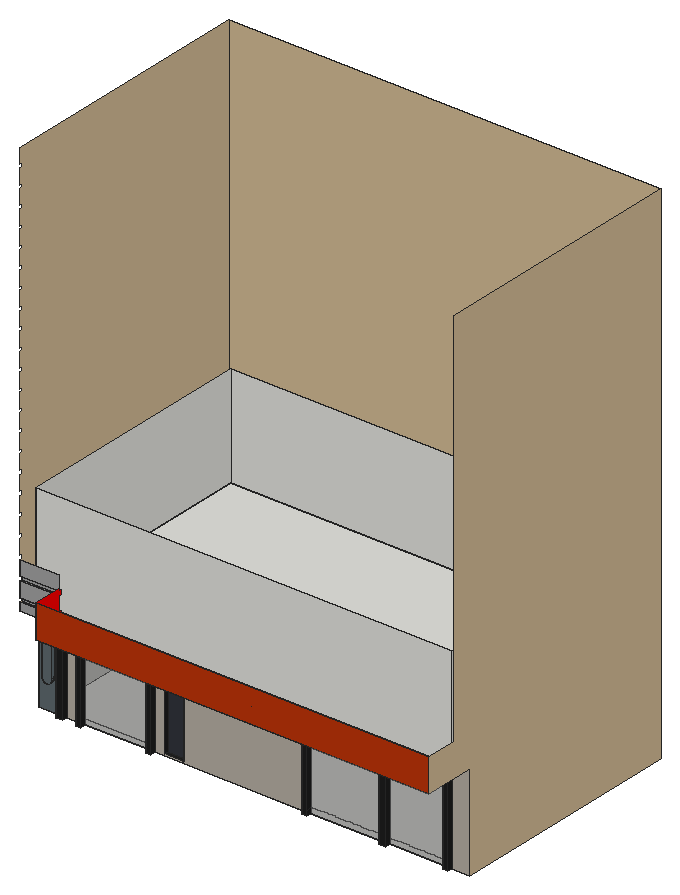
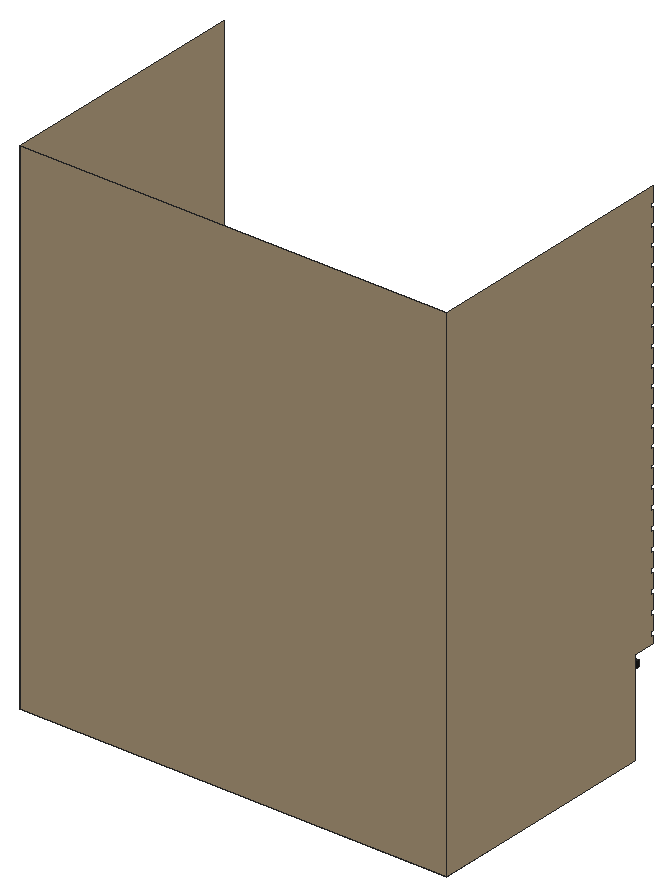
# SketchUp Ruby script. Lengths in inches.
U = 1.inch
M = Sketchup.active_model
def pt(a) = Geom::Point3d.new(a.map { |v| v * U })
def face(e, loops, mat)
  f = e.add_face(loops[0].map { |a| pt(a) })
  loops[1..].each { |l| e.add_face(l.map { |a| pt(a) }).erase! }
  f.material = f.back_material = mat if mat
  f
end
# faces: each face lists its corners as indices into pts; further lists are holes
def faces(e, pts, list, mat = nil) = list.each { |f| face(e, (f[0].is_a?(Array) ? f : [f]).map { |l| l.map { |i| pts[i] } }, mat) }
# xy, xz, yz: faces in a plane at the given z, y or x. An outline is a flat list of corners, or four numbers for a rectangle; further outlines are holes
def ring(l) = l.size == 4 ? [[l[0], l[1]], [l[2], l[1]], [l[2], l[3]], [l[0], l[3]]] : l.each_slice(2).to_a
def flat(e, list, mat, &to3) = list.each { |f| face(e, (f[0].is_a?(Array) ? f : [f]).map { |l| ring(l).map { |u, v| to3.(u, v) } }, mat) }
def xy(e, z, list, mat = nil) = flat(e, list, mat) { |x, y| [x, y, z] }
def xz(e, y, list, mat = nil) = flat(e, list, mat) { |x, z| [x, y, z] }
def yz(e, x, list, mat = nil) = flat(e, list, mat) { |y, z| [x, y, z] }
def lines(e, pts, list) = list.each { |a, b| e.add_line(pt(pts[a]), pt(pts[b])) }
# prism: a flat outline (further loops are holes) pulled along v
def prism(e, loops, v, mat = nil)
  f = face(e, loops, mat); d = Geom::Vector3d.new(v.map { |x| x * U })
  f.pushpull(f.normal.samedirection?(d) ? d.length : -d.length)
end
def box(e, o, s, mat = nil) = prism(e, [[o, [o[0] + s[0], o[1], o[2]], [o[0] + s[0], o[1] + s[1], o[2]], [o[0], o[1] + s[1], o[2]]]], [0, 0, s[2]], mat)
def at(x, y, z, deg = 0) = Geom::Transformation.translation(pt([x, y, z])) * Geom::Transformation.rotation(ORIGIN, Z_AXIS, deg.degrees)
def axes(o, x, y, z) = Geom::Transformation.new([*x, 0, *y, 0, *z, 0, *pt(o).to_a, 1])
def part(name) = M.definitions.add(name)
# library, detail: a bought-in or finely detailed component or shape, given as its bounding box
def library(name, o, s) = part(name).tap { |d| box(d.entities, o, s) }
def detail(e, o, s) = box(e.add_group.entities, o, s)
def put(e, d, t, mat = nil) = e.add_instance(d, t).tap { |i| i.material = mat if mat }
def group(e, t, mat = nil) = e.add_group.tap { |g| g.transformation = t; g.material = mat if mat }.entities
root = M.entities
M.materials.add("[0020_Red]").color = [255, 0, 0]
M.materials.add("[Blacktop New]").color = [30, 30, 30]
M.materials.add("[Formica Beige]").color = [211, 187, 149]
M.materials.add("[Formica Laminate Dark]").color = [50, 53, 60]
M.materials.add("[Formica Speckled Grey]").color = [94, 105, 111]
M.materials.add("[Modern Siding]1").color = [191, 52, 9]
M.materials.add("[Pavers Flagstone Gray]").color = [162, 162, 162]
M.materials.add("[Stone Masonry Multi]").color = [182, 175, 164]
M.materials.add("[Translucent Glass Gray]").color = [128, 128, 128]
M.materials["[Translucent Glass Gray]"].alpha = 0.5
M.materials.add("[Wood Veneer 01]").color = [120, 70, 37]
xy(root,0,[[[48.29,57,48.29,63,0,63,0,342.4375,506.625,342.4375,506.625,63,485.22,63,485.22,57,479.22,57,479.22,63,411.96,63,411.96,57,404.66,57,404.66,63,320.21,63,320.21,57,314.21,57,314.21,63,136.16,63,136.16,57,130.16,57,130.16,63,54.29,63,54.29,57],[9,72,497.625,333.4375]],[24.71,57,33.0625,63],[9,72,497.625,333.4375]])
xy(root,1.93,[[147.93,63,170.18,68.3125]],"[Blacktop New]")
xy(root,97.39,[[0,57,24.71,63]],"[Blacktop New]")
xy(root,99.6875,[[320.21,57,404.66,63],[411.96,57,479.22,63]],"[Blacktop New]")
xy(root,103.25,[[54.29,57,130.16,63]],"[Blacktop New]")
xy(root,105.58,[[0,57,33.0625,63]],"[Blacktop New]")
xy(root,105.6875,[[314.21,57,485.22,63]])
xy(root,109.25,[[48.29,57,136.16,63]],"[Blacktop New]")
xy(root,110.37,[[147.93,63,170.18,68.3125]],"[Blacktop New]")
xy(root,112.65,[[45.0625,3,45.0625,36,0,36,0,63,506.625,63,506.625,3]],"[Wood Veneer 01]")
xy(root,120,[[9,48,497.625,333.4375]])
xy(root,121.8125,[[0,36,45.0625,39]],"[Pavers Flagstone Gray]")
xy(root,126.82,[[0,36,45.0625,39]],"[Pavers Flagstone Gray]")
xy(root,144.1875,[[0,36,45.0625,39]],"[Pavers Flagstone Gray]")
xy(root,149.2,[[0,36,45.0625,39]],"[Pavers Flagstone Gray]")
xz(root,3,[[45.0625,112.65,506.625,151.96]],"[Modern Siding]1")
xz(root,36,[[0,112.65,45.0625,121.8125],[0,126.82,45.0625,144.1875],[0,149.2,45.0625,166.5625]],"[Pavers Flagstone Gray]")
xz(root,39,[[0,121.8125,45.0625,126.82],[0,144.1875,45.0625,149.2]],"[Pavers Flagstone Gray]")
xz(root,48,[[9,120,497.625,240]])
xz(root,57,[[24.71,0,33.0625,0,33.0625,105.58,0,105.58,0,97.39,24.71,97.39],[48.29,0,54.29,0,54.29,103.25,130.16,103.25,130.16,0,136.16,0,136.16,109.25,48.29,109.25],[314.21,0,320.21,0,320.21,99.6875,479.22,99.6875,479.22,0,485.22,0,485.22,105.6875,314.21,105.6875],[404.66,0,411.96,99.6875]],"[Blacktop New]")
xz(root,60,[[11.84,29.86,13.68,30.13,15.37,30.92,16.76,32.17,17.72,33.76,18.12,35.28,18.12,84,17.9,85.63,17.28,87.14,16.28,88.44,14.98,89.44,13.46,90.07,11.84,90.28,10.21,90.07,8.7,89.44,7.4,88.44,6.4,87.14,5.77,85.63,5.56,84,5.56,35.28,5.95,33.76,6.92,32.17,8.3,30.92,9.99,30.13]],"[Formica Speckled Grey]")
xz(root,63,[[24.71,0,24.71,97.39,0,97.39,0,105.58,33.0625,105.58,33.0625,0],[5.56,35.28,5.56,37.43,5.48,35.57],[18.12,35.28,18.19,35.57,18.12,37.43]])
xz(root,63,[[[0,0,24.71,97.39],[11.84,29.86,9.99,30.13,8.3,30.92,6.92,32.17,5.95,33.76,5.56,35.28,5.48,35.57,5.56,37.43,5.56,84,5.77,85.63,6.4,87.14,7.4,88.44,8.7,89.44,10.21,90.07,11.84,90.28,13.46,90.07,14.98,89.44,16.28,88.44,17.28,87.14,17.9,85.63,18.12,84,18.12,37.43,18.19,35.57,18.12,35.28,17.72,33.76,16.76,32.17,15.37,30.92,13.68,30.13]]],"[Formica Speckled Grey]")
xz(root,63,[[[33.0625,0,48.29,0,48.29,109.25,136.16,109.25,136.16,0,314.21,0,314.21,105.6875,485.22,105.6875,485.22,0,506.625,0,506.625,112.65,0,112.65,0,105.58,33.0625,105.58],[147.93,1.93,170.18,110.37]]],"[Stone Masonry Multi]")
xz(root,63,[[54.29,0,130.16,103.25],[320.21,0,404.66,99.6875],[411.96,0,479.22,99.6875]],"[Translucent Glass Gray]")
xz(root,68.3125,[[147.93,1.93,170.18,110.37]],"[Formica Laminate Dark]")
xz(root,333.4375,[[9,0,497.625,120],[9,120,497.625,240]])
xz(root,342.4375,[[0,0,506.625,600]],"[Formica Beige]")
yz(root,0,[[57,97.39,63,105.58]],"[Blacktop New]")
yz(root,0,[[63,0,63,112.65,36,112.65,36,121.8125,39,121.8125,39,126.82,36,126.82,36,144.1875,39,144.1875,39,149.2,36,149.2,36,166.5625,39,166.5625,39,171.57,36,171.57,36,188.9375,39,188.9375,39,193.95,36,193.95,36,211.3125,39,211.3125,39,216.32,36,216.32,36,233.6875,39,233.6875,39,238.7,36,238.7,36,256.0625,39,256.0625,39,261.07,36,261.07,36,278.4375,39,278.4375,39,282.51,36,282.51,36,299.875,39,299.875,39,303.95,36,303.95,36,321.3125,39,321.3125,39,325.39,36,325.39,36,342.75,39,342.75,39,346.82,36,346.82,36,364.1875,39,364.1875,39,368.26,36,368.26,36,385.625,39,385.625,39,389.7,36,389.7,36,407.0625,39,407.0625,39,411.14,36,411.14,36,428.5,39,428.5,39,432.57,36,432.57,36,449.9375,39,449.9375,39,454.01,36,454.01,36,471.375,39,471.375,39,475.45,36,475.45,36,492.8125,39,492.8125,39,496.89,36,496.89,36,514.25,39,514.25,39,518.32,36,518.32,36,535.6875,39,535.6875,39,539.76,36,539.76,36,557.125,39,557.125,39,561.2,36,561.2,36,578.5625,39,578.5625,39,582.64,36,582.64,36,600,342.4375,600,342.4375,0]],"[Formica Beige]")
yz(root,5.56,[[60,35.28,63,37.43],[60,37.43,63,84]],"[Formica Speckled Grey]")
yz(root,9,[[72,0,333.4375,120],[48,120,333.4375,240]])
yz(root,18.12,[[60,35.28,63,37.43],[60,37.43,63,84]],"[Formica Speckled Grey]")
yz(root,24.71,[[57,0,63,97.39]],"[Blacktop New]")
yz(root,33.0625,[[57,0,63,105.58]],"[Blacktop New]")
yz(root,45.0625,[[3,112.65,3,151.96,36,151.96,36,149.2,39,149.2,39,144.1875,36,144.1875,36,126.82,39,126.82,39,121.8125,36,121.8125,36,112.65]],"[0020_Red]")
yz(root,48.29,[[57,0,63,109.25]],"[Blacktop New]")
yz(root,54.29,[[57,0,63,103.25]],"[Blacktop New]")
yz(root,130.16,[[57,0,63,103.25]],"[Blacktop New]")
yz(root,136.16,[[57,0,63,109.25]],"[Blacktop New]")
yz(root,147.93,[[63,1.93,68.3125,110.37]],"[Blacktop New]")
yz(root,170.18,[[63,1.93,68.3125,110.37]],"[Blacktop New]")
yz(root,314.21,[[57,0,63,105.6875]],"[Blacktop New]")
yz(root,320.21,[[57,0,63,6],[57,6,63,99.6875]],"[Blacktop New]")
yz(root,404.66,[[57,0,63,99.6875]],"[Blacktop New]")
yz(root,411.96,[[57,0,63,99.6875]],"[Blacktop New]")
yz(root,479.22,[[57,0,63,6]])
yz(root,479.22,[[57,6,63,99.6875]],"[Blacktop New]")
yz(root,485.22,[[57,0,63,105.6875]],"[Blacktop New]")
yz(root,497.625,[[72,0,333.4375,120],[48,120,333.4375,240]])
yz(root,506.625,[[63,0,342.4375,0,342.4375,600,39,600,39,151.96,3,151.96,3,112.65,63,112.65]],"[Formica Beige]")
p = [[9.99,63,30.13],[11.84,63,29.86],[11.84,60,29.86],[9.99,60,30.13],[13.68,63,30.13],[13.68,60,30.13],
  [8.3,63,30.92],[8.3,60,30.92],[15.37,63,30.92],[15.37,60,30.92],[6.92,63,32.17],[6.92,60,32.17],
  [16.76,63,32.17],[16.76,60,32.17],[5.95,63,33.76],[5.95,60,33.76],[17.72,63,33.76],[17.72,60,33.76],
  [5.56,63,35.28],[5.56,60,35.28],[18.12,63,35.28],[18.12,60,35.28],[5.77,63,85.63],[5.56,63,84],
  [5.56,60,84],[5.77,60,85.63],[18.12,63,84],[17.9,63,85.63],[17.9,60,85.63],[18.12,60,84],
  [6.4,63,87.14],[6.4,60,87.14],[17.28,63,87.14],[17.28,60,87.14],[7.4,63,88.44],[7.4,60,88.44],
  [16.28,63,88.44],[16.28,60,88.44],[8.7,63,89.44],[8.7,60,89.44],[14.98,63,89.44],[14.98,60,89.44],
  [10.21,63,90.07],[10.21,60,90.07],[13.46,63,90.07],[13.46,60,90.07],[11.84,63,90.28],[11.84,60,90.28],
  [297.58,3,131.5],[297.58,3,131.43]]
faces(root,p,[[0,1,2,3],[1,4,5,2],[6,0,3,7],[4,8,9,5],[10,6,7,11],[8,12,13,9],[14,10,11,15],[12,16,17,13],
  [18,14,15,19],[16,20,21,17],[22,23,24,25],[26,27,28,29],[30,22,25,31],[27,32,33,28],[34,30,31,35],[32,36,37,33],
  [38,34,35,39],[36,40,41,37],[42,38,39,43],[40,44,45,41],[46,42,43,47],[44,46,47,45]],"[Formica Speckled Grey]")
lines(root,p,[[48,49]])
